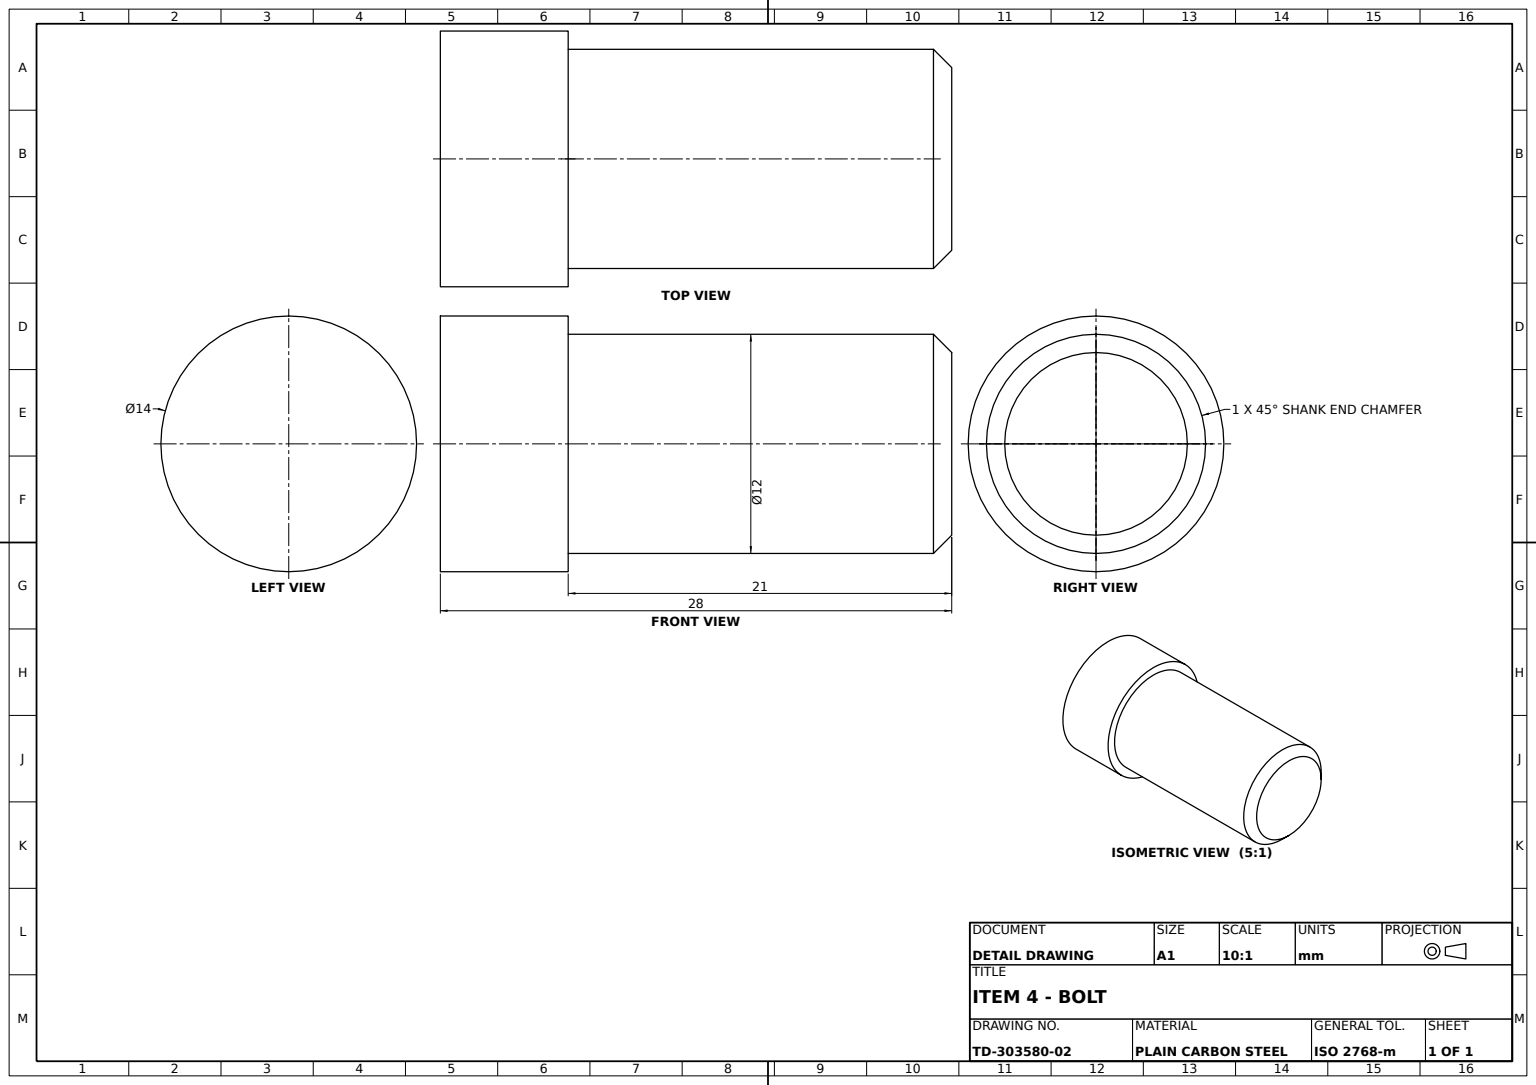
ISO-10303-21;
HEADER;
FILE_DESCRIPTION((''),'2;1');
FILE_NAME('','',(''),(''),'','','');
FILE_SCHEMA(('AUTOMOTIVE_DESIGN'));
ENDSEC;
DATA;
#1=APPLICATION_CONTEXT('');
#2=PRODUCT_CONTEXT('',#1,'mechanical');
#3=PRODUCT('','','',(#2));
#4=PRODUCT_DEFINITION_FORMATION('','',#3);
#5=PRODUCT_DEFINITION_CONTEXT('',#1,'design');
#6=PRODUCT_DEFINITION('','',#4,#5);
#7=PRODUCT_DEFINITION_SHAPE('','',#6);
#8=(LENGTH_UNIT()NAMED_UNIT(*)SI_UNIT(.MILLI.,.METRE.));
#9=(NAMED_UNIT(*)PLANE_ANGLE_UNIT()SI_UNIT($,.RADIAN.));
#10=(NAMED_UNIT(*)SI_UNIT($,.STERADIAN.)SOLID_ANGLE_UNIT());
#11=UNCERTAINTY_MEASURE_WITH_UNIT(LENGTH_MEASURE(1.E-05),#8,'distance_accuracy_value','');
#12=(GEOMETRIC_REPRESENTATION_CONTEXT(3)GLOBAL_UNCERTAINTY_ASSIGNED_CONTEXT((#11))GLOBAL_UNIT_ASSIGNED_CONTEXT((#8,#9,#10))REPRESENTATION_CONTEXT('',''));
#13=CARTESIAN_POINT('',(-21.,-6.,0.));
#14=VERTEX_POINT('',#13);
#15=CARTESIAN_POINT('',(-1.,-6.,0.));
#16=VERTEX_POINT('',#15);
#17=CARTESIAN_POINT('',(0.,-6.,0.));
#18=DIRECTION('',(1.,0.,0.));
#19=VECTOR('',#18,1000.);
#20=LINE('',#17,#19);
#21=EDGE_CURVE('',#14,#16,#20,.T.);
#22=ORIENTED_EDGE('',*,*,#21,.T.);
#23=CARTESIAN_POINT('',(-1.,6.,0.));
#24=VERTEX_POINT('',#23);
#25=CARTESIAN_POINT('',(-1.,0.,0.));
#26=DIRECTION('',(-1.,0.,0.));
#27=DIRECTION('',(0.,1.,0.));
#28=AXIS2_PLACEMENT_3D('',#25,#26,#27);
#29=CIRCLE('',#28,6.);
#30=EDGE_CURVE('',#16,#24,#29,.T.);
#31=ORIENTED_EDGE('',*,*,#30,.T.);
#32=CARTESIAN_POINT('',(-21.,6.,0.));
#33=VERTEX_POINT('',#32);
#34=CARTESIAN_POINT('',(0.,6.,0.));
#35=LINE('',#34,#19);
#36=EDGE_CURVE('',#33,#24,#35,.T.);
#37=ORIENTED_EDGE('',*,*,#36,.F.);
#38=CARTESIAN_POINT('',(-21.,0.,0.));
#39=AXIS2_PLACEMENT_3D('',#38,#18,#27);
#40=CIRCLE('',#39,6.);
#41=EDGE_CURVE('',#33,#14,#40,.T.);
#42=ORIENTED_EDGE('',*,*,#41,.T.);
#43=EDGE_LOOP('',(#22,#31,#37,#42));
#44=FACE_OUTER_BOUND('',#43,.T.);
#45=CARTESIAN_POINT('',(0.,0.,0.));
#46=AXIS2_PLACEMENT_3D('',#45,#18,#27);
#47=CYLINDRICAL_SURFACE('',#46,6.);
#48=ADVANCED_FACE('',(#44),#47,.T.);
#49=CARTESIAN_POINT('',(-28.,7.,0.));
#50=VERTEX_POINT('',#49);
#51=CARTESIAN_POINT('',(-28.,-7.,0.));
#52=VERTEX_POINT('',#51);
#53=CARTESIAN_POINT('',(-28.,0.,0.));
#54=AXIS2_PLACEMENT_3D('',#53,#18,#27);
#55=CIRCLE('',#54,7.);
#56=EDGE_CURVE('',#50,#52,#55,.T.);
#57=ORIENTED_EDGE('',*,*,#56,.F.);
#58=EDGE_CURVE('',#52,#50,#55,.T.);
#59=ORIENTED_EDGE('',*,*,#58,.F.);
#60=EDGE_LOOP('',(#57,#59));
#61=FACE_OUTER_BOUND('',#60,.T.);
#62=DIRECTION('',(0.,-1.,0.));
#63=AXIS2_PLACEMENT_3D('',#49,#26,#62);
#64=PLANE('',#63);
#65=ADVANCED_FACE('',(#61),#64,.T.);
#66=CARTESIAN_POINT('',(0.,-5.,0.));
#67=VERTEX_POINT('',#66);
#68=CARTESIAN_POINT('',(0.,5.,0.));
#69=VERTEX_POINT('',#68);
#70=CIRCLE('',#46,5.);
#71=EDGE_CURVE('',#67,#69,#70,.T.);
#72=ORIENTED_EDGE('',*,*,#71,.T.);
#73=EDGE_CURVE('',#69,#67,#70,.T.);
#74=ORIENTED_EDGE('',*,*,#73,.T.);
#75=EDGE_LOOP('',(#72,#74));
#76=FACE_OUTER_BOUND('',#75,.T.);
#77=PLANE('',#46);
#78=ADVANCED_FACE('',(#76),#77,.T.);
#79=CARTESIAN_POINT('',(-21.,7.,0.));
#80=VERTEX_POINT('',#79);
#81=CARTESIAN_POINT('',(-21.,-7.,0.));
#82=VERTEX_POINT('',#81);
#83=CIRCLE('',#39,7.);
#84=EDGE_CURVE('',#80,#82,#83,.T.);
#85=ORIENTED_EDGE('',*,*,#84,.T.);
#86=EDGE_CURVE('',#82,#80,#83,.T.);
#87=ORIENTED_EDGE('',*,*,#86,.T.);
#88=EDGE_LOOP('',(#85,#87));
#89=FACE_OUTER_BOUND('',#88,.T.);
#90=ORIENTED_EDGE('',*,*,#41,.F.);
#91=EDGE_CURVE('',#14,#33,#40,.T.);
#92=ORIENTED_EDGE('',*,*,#91,.F.);
#93=EDGE_LOOP('',(#90,#92));
#94=FACE_BOUND('',#93,.T.);
#95=AXIS2_PLACEMENT_3D('',#32,#18,#27);
#96=PLANE('',#95);
#97=ADVANCED_FACE('',(#89,#94),#96,.T.);
#98=ORIENTED_EDGE('',*,*,#30,.F.);
#99=DIRECTION('',(-0.707106781,-0.707106781,0.));
#100=VECTOR('',#99,1000.);
#101=LINE('',#66,#100);
#102=EDGE_CURVE('',#67,#16,#101,.T.);
#103=ORIENTED_EDGE('',*,*,#102,.F.);
#104=ORIENTED_EDGE('',*,*,#73,.F.);
#105=DIRECTION('',(-0.707106781,0.707106781,0.));
#106=VECTOR('',#105,1000.);
#107=LINE('',#68,#106);
#108=EDGE_CURVE('',#69,#24,#107,.T.);
#109=ORIENTED_EDGE('',*,*,#108,.T.);
#110=EDGE_LOOP('',(#98,#103,#104,#109));
#111=FACE_OUTER_BOUND('',#110,.T.);
#112=AXIS2_PLACEMENT_3D('',#45,#26,#62);
#113=CONICAL_SURFACE('',#112,5.,0.785398163);
#114=ADVANCED_FACE('',(#111),#113,.T.);
#115=ORIENTED_EDGE('',*,*,#84,.F.);
#116=CARTESIAN_POINT('',(0.,7.,0.));
#117=LINE('',#116,#19);
#118=EDGE_CURVE('',#50,#80,#117,.T.);
#119=ORIENTED_EDGE('',*,*,#118,.F.);
#120=ORIENTED_EDGE('',*,*,#56,.T.);
#121=CARTESIAN_POINT('',(0.,-7.,0.));
#122=LINE('',#121,#19);
#123=EDGE_CURVE('',#52,#82,#122,.T.);
#124=ORIENTED_EDGE('',*,*,#123,.T.);
#125=EDGE_LOOP('',(#115,#119,#120,#124));
#126=FACE_OUTER_BOUND('',#125,.T.);
#127=CYLINDRICAL_SURFACE('',#46,7.);
#128=ADVANCED_FACE('',(#126),#127,.T.);
#129=ORIENTED_EDGE('',*,*,#108,.F.);
#130=ORIENTED_EDGE('',*,*,#71,.F.);
#131=ORIENTED_EDGE('',*,*,#102,.T.);
#132=EDGE_CURVE('',#24,#16,#29,.T.);
#133=ORIENTED_EDGE('',*,*,#132,.F.);
#134=EDGE_LOOP('',(#129,#130,#131,#133));
#135=FACE_OUTER_BOUND('',#134,.T.);
#136=ADVANCED_FACE('',(#135),#113,.T.);
#137=ORIENTED_EDGE('',*,*,#91,.T.);
#138=ORIENTED_EDGE('',*,*,#36,.T.);
#139=ORIENTED_EDGE('',*,*,#132,.T.);
#140=ORIENTED_EDGE('',*,*,#21,.F.);
#141=EDGE_LOOP('',(#137,#138,#139,#140));
#142=FACE_OUTER_BOUND('',#141,.T.);
#143=ADVANCED_FACE('',(#142),#47,.T.);
#144=ORIENTED_EDGE('',*,*,#58,.T.);
#145=ORIENTED_EDGE('',*,*,#118,.T.);
#146=ORIENTED_EDGE('',*,*,#86,.F.);
#147=ORIENTED_EDGE('',*,*,#123,.F.);
#148=EDGE_LOOP('',(#144,#145,#146,#147));
#149=FACE_OUTER_BOUND('',#148,.T.);
#150=ADVANCED_FACE('',(#149),#127,.T.);
#151=CLOSED_SHELL('',(#48,#65,#78,#97,#114,#128,#136,#143,#150));
#152=MANIFOLD_SOLID_BREP('',#151);
#153=ADVANCED_BREP_SHAPE_REPRESENTATION('',(#152),#12);
#154=SHAPE_DEFINITION_REPRESENTATION(#7,#153);
ENDSEC;
END-ISO-10303-21;
